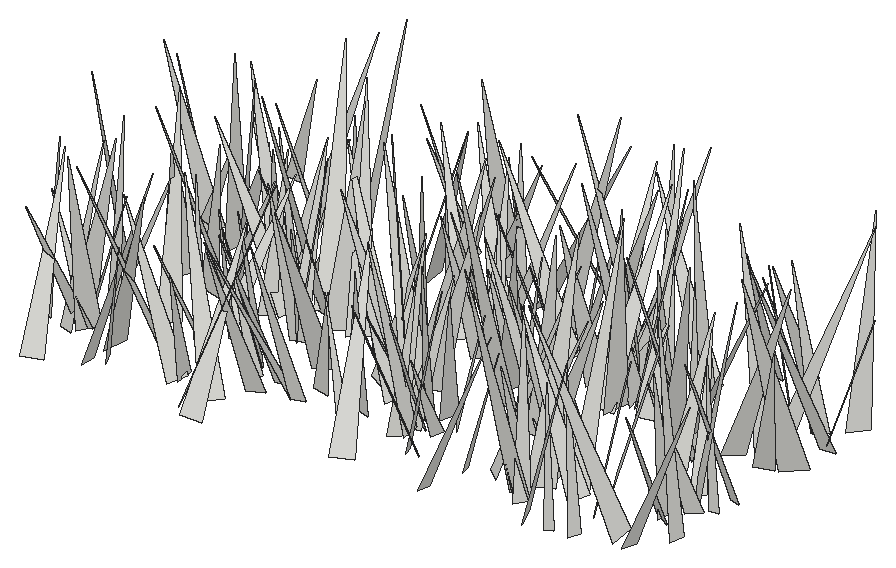
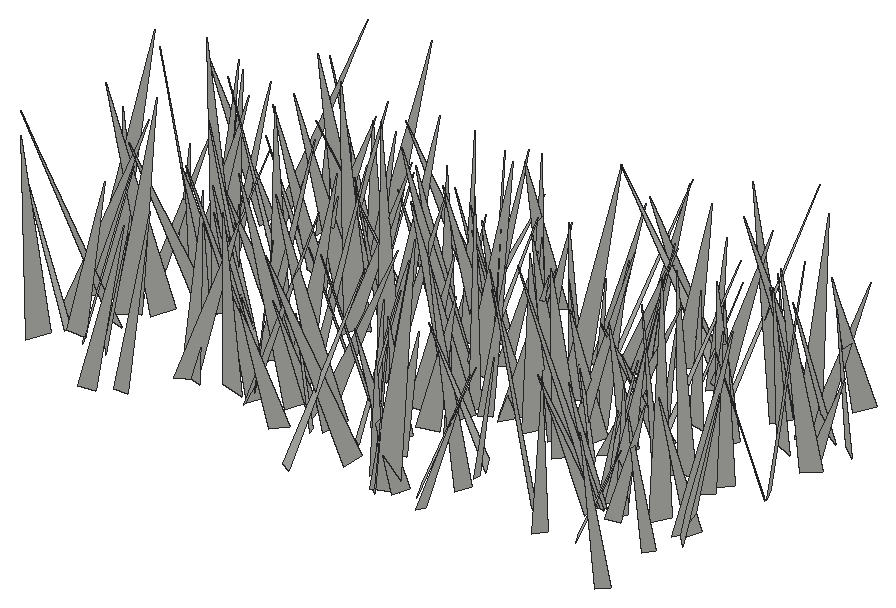
# SketchUp Ruby script. Lengths in inches.
U = 1.inch
M = Sketchup.active_model
def pt(a) = Geom::Point3d.new(a.map { |v| v * U })
def face(e, loops, mat)
  f = e.add_face(loops[0].map { |a| pt(a) })
  loops[1..].each { |l| e.add_face(l.map { |a| pt(a) }).erase! }
  f.material = f.back_material = mat if mat
  f
end
# faces: each face lists its corners as indices into pts; further lists are holes
def faces(e, pts, list, mat = nil) = list.each { |f| face(e, (f[0].is_a?(Array) ? f : [f]).map { |l| l.map { |i| pts[i] } }, mat) }
# xy, xz, yz: faces in a plane at the given z, y or x. An outline is a flat list of corners, or four numbers for a rectangle; further outlines are holes
def ring(l) = l.size == 4 ? [[l[0], l[1]], [l[2], l[1]], [l[2], l[3]], [l[0], l[3]]] : l.each_slice(2).to_a
def flat(e, list, mat, &to3) = list.each { |f| face(e, (f[0].is_a?(Array) ? f : [f]).map { |l| ring(l).map { |u, v| to3.(u, v) } }, mat) }
def xy(e, z, list, mat = nil) = flat(e, list, mat) { |x, y| [x, y, z] }
def xz(e, y, list, mat = nil) = flat(e, list, mat) { |x, z| [x, y, z] }
def yz(e, x, list, mat = nil) = flat(e, list, mat) { |y, z| [x, y, z] }
def lines(e, pts, list) = list.each { |a, b| e.add_line(pt(pts[a]), pt(pts[b])) }
# prism: a flat outline (further loops are holes) pulled along v
def prism(e, loops, v, mat = nil)
  f = face(e, loops, mat); d = Geom::Vector3d.new(v.map { |x| x * U })
  f.pushpull(f.normal.samedirection?(d) ? d.length : -d.length)
end
def box(e, o, s, mat = nil) = prism(e, [[o, [o[0] + s[0], o[1], o[2]], [o[0] + s[0], o[1] + s[1], o[2]], [o[0], o[1] + s[1], o[2]]]], [0, 0, s[2]], mat)
def at(x, y, z, deg = 0) = Geom::Transformation.translation(pt([x, y, z])) * Geom::Transformation.rotation(ORIGIN, Z_AXIS, deg.degrees)
def axes(o, x, y, z) = Geom::Transformation.new([*x, 0, *y, 0, *z, 0, *pt(o).to_a, 1])
def part(name) = M.definitions.add(name)
# library, detail: a bought-in or finely detailed component or shape, given as its bounding box
def library(name, o, s) = part(name).tap { |d| box(d.entities, o, s) }
def detail(e, o, s) = box(e.add_group.entities, o, s)
def put(e, d, t, mat = nil) = e.add_instance(d, t).tap { |i| i.material = mat if mat }
def group(e, t, mat = nil) = e.add_group.tap { |g| g.transformation = t; g.material = mat if mat }.entities
root = M.entities
c1 = part("fur_instance\#9")
p = [[0.8125,0,1.79],[0.67,-0.02,1.48],[0,-0.11,0],[0,0.11,0]]
faces(c1.entities,p,[[0,1,2,3]])
put(root,c1,axes([517.29,201.38,-21.66],[-1.69129,6.09931,0.73665],[6.01995,1.79783,-1.06428],[1.22654,-0.41345,6.23934]))
put(root,c1,axes([513.87,205.09,-21.66],[4.34393,-1.36952,0.92271],[-1.07858,-4.31928,-1.3331],[-1.25046,-1.03195,4.35524]))
put(root,c1,axes([508.99,203.98,-21.66],[3.83115,1.46002,1.29175],[1.69697,-3.89964,-0.62537],[-0.95945,-1.06731,4.05194]))
put(root,c1,axes([512.04,206.01,-21.66],[-5.96811,-4.81477,0.42538],[-4.75156,5.96808,0.88657],[0.88638,-0.42578,7.61672]))
put(root,c1,axes([505.45,201.28,-21.66],[-4.47188,4.60163,0.40246],[4.4512,4.44255,-1.33612],[1.23441,0.65071,6.27595]))
put(root,c1,axes([508.34,205.5,-21.66],[6.88515,-2.28469,0.18682],[-2.24647,-6.84269,-0.88939],[-0.45618,-0.78602,7.19959]))
put(root,c1,axes([505.62,206.01,-21.66],[0.74185,-5.118,0.35857],[-5.01336,-0.80012,-1.04825],[-1.09027,0.19676,5.06413]))
put(root,c1,axes([508.27,203.01,-21.66],[6.55283,1.12937,1.12544],[0.97488,-6.60494,0.95181],[-1.26162,0.76214,6.58096]))
put(root,c1,axes([518.27,206.27,-21.66],[1.50349,-5.86365,0.5049],[-5.82358,-1.55753,-0.74685],[-0.85041,0.2992,6.00709]))
put(root,c1,axes([540.07,204.38,-21.66],[5.73054,2.09287,1.0832],[2.24178,-5.71944,-0.8093],[-0.7265,-1.14039,6.04684]))
put(root,c1,axes([513.75,204.54,-21.66],[-5.32926,2.77314,1.19327],[2.9808,5.21718,1.1879],[0.47858,-1.6143,5.88899]))
put(root,c1,axes([505.83,206.11,-21.66],[4.78165,-4.93816,1.39024],[-4.88475,-4.96331,-0.82896],[-1.56762,0.40313,6.82367]))
put(root,c1,axes([533.17,203.42,-21.66],[5.62442,0.34622,0.61815],[0.22701,-5.5658,1.05184],[-0.67115,1.01884,5.53603]))
put(root,c1,axes([515.5625,202.65,-21.66],[6.75975,3.62956,0.52461],[3.54067,-6.74583,1.04905],[-0.95528,0.68056,7.60048]))
put(root,c1,axes([519.79,207.6,-21.66],[-4.86076,-4.47494,0.06756],[-4.36579,4.76306,1.38194],[0.98465,-0.972,6.46083]))
put(root,c1,axes([516.86,203.93,-21.66],[-4.60264,5.20733,0.96805],[5.29634,4.53648,0.77902],[0.04773,-1.24166,6.90606]))
put(root,c1,axes([545.83,206.21,-21.66],[-8.03194,-0.35365,0.82088],[-0.22203,7.97883,1.26494],[0.86581,-1.23463,7.93959]))
put(root,c1,axes([538.1,206.26,-21.66],[-1.48143,-7.59825,2.03928],[-7.84224,1.26126,-0.99758],[-0.62555,2.18232,7.67677]))
put(root,c1,axes([526.82,204.11,-21.66],[-4.67353,1.04438,0.03845],[1.02272,4.60667,-0.8165],[0.21505,0.78861,4.71868]))
put(root,c1,axes([543.59,204.51,-21.66],[-4.82421,0.67017,1.12309],[0.52178,4.9221,-0.69578],[1.19925,0.5543,4.82058]))
put(root,c1,axes([542.04,204.11,-21.66],[0.68638,4.30492,0.85677],[4.11958,-0.93113,1.37825],[-1.51508,-0.58153,4.13569]))
put(root,c1,axes([527.17,203.23,-21.66],[-3.85678,5.81728,0.33644],[5.7739,3.8696,-0.71896],[0.78484,0.11882,6.94252]))
put(root,c1,axes([530.33,206.41,-21.66],[-3.6362,-3.51378,0.23491],[-3.4583,3.49912,-1.19165],[-0.6648,1.01649,4.91412]))
put(root,c1,axes([520.81,207.0625,-21.66],[-0.18696,-5.47828,1.21386],[-5.53827,-0.01495,-0.92048],[-0.90141,1.22808,5.40363]))
put(root,c1,axes([546.94,205.55,-21.66],[5.55155,-0.72144,0.45458],[-0.77671,-5.51397,0.73462],[-0.35191,0.78896,5.54982]))
put(root,c1,axes([513.29,207.97,-21.66],[-3.4189,-2.83051,0.24342],[-2.77437,3.40847,0.66713],[0.61145,-0.36118,4.38812]))
put(root,c1,axes([537.24,207.9375,-21.66],[4.28198,-1.79299,1.3249],[-1.43721,-4.41332,-1.32759],[-1.70429,-0.78312,4.44833]))
put(root,c1,axes([537.33,206.62,-21.66],[-3.51582,-2.14374,0.80605],[-2.26912,3.46073,-0.69338],[0.31056,1.01688,4.05904]))
put(root,c1,axes([524.47,208.31,-21.66],[-0.27546,-6.0552,1.07535],[-6.00995,0.49341,1.23885],[1.30474,0.99438,5.93351]))
put(root,c1,axes([502.96,205.89,-21.66],[2.73063,4.59292,1.67983],[4.59916,-3.06583,0.90635],[-1.66266,-0.93747,5.2659]))
put(root,c1,axes([538.68,205.75,-21.66],[-5.6137,1.8249,1.28834],[1.63706,5.7317,-0.98561],[1.51991,0.56669,5.82001]))
put(root,c1,axes([517.29,207.57,-21.66],[-3.50463,1.38607,1.3282],[1.66931,3.56562,0.68373],[0.94799,-1.15452,3.70623]))
put(root,c1,axes([504.88,205.18,-21.66],[2.36342,5.34352,0.74133],[5.25737,-2.46286,0.99138],[-1.20944,-0.26392,5.75813]))
put(root,c1,axes([504.83,207.71,-21.66],[4.88196,1.64498,0.71636],[1.77456,-4.73338,-1.22423],[-0.26474,-1.39349,5.00407]))
put(root,c1,axes([546.35,209.35,-21.66],[-1.70648,-4.83175,0.15849],[-4.67215,1.69151,1.26205],[1.24174,-0.27565,4.96639]))
put(root,c1,axes([518.73,207.97,-21.66],[-1.8038,-4.78632,0.84713],[-4.75617,1.55162,-1.36069],[-1.00264,1.25053,4.93062]))
put(root,c1,axes([529.75,208.97,-21.66],[2.79879,-2.29313,0.37979],[-2.08936,-2.74248,-1.16161],[-1.01846,-0.6755,3.42672]))
put(root,c1,axes([533.73,206.61,-21.66],[3.61402,1.40651,0.81578],[1.29809,-3.69316,0.61679],[-0.97915,0.29527,3.8287]))
put(root,c1,axes([528.375,208.27,-21.66],[-6.31827,-0.38458,1.65434],[-0.20418,6.49842,0.73085],[1.68614,-0.65417,6.28763]))
put(root,c1,axes([521.23,208.6875,-21.66],[0.93641,-4.49496,0.58968],[-4.44892,-0.79539,1.00188],[0.87152,0.76939,4.48082]))
put(root,c1,axes([529.68,206.29,-21.66],[4.20978,2.5999,1.29958],[2.36123,-4.39284,1.13935],[-1.69498,0.33775,4.81493]))
put(root,c1,axes([528.42,209.24,-21.66],[-1.9531,-3.93926,0.49775],[-3.87343,2.01224,0.72636],[0.87298,0.11511,4.33645]))
put(root,c1,axes([516.32,209.37,-21.66],[-3.7934,-3.57067,0.95546],[-3.47781,3.9116,0.81037],[1.25196,0.04698,5.14615]))
put(root,c1,axes([541.03,208.16,-21.66],[-5.49496,2.98551,0.84144],[3.09795,5.36781,1.18541],[0.15494,-1.44541,6.14025]))
put(root,c1,axes([528.74,209.5,-21.66],[-1.97091,-5.99186,1.73382],[-5.97714,2.33419,1.27215],[1.7839,1.20092,6.17807]))
put(root,c1,axes([503.9,208.01,-21.66],[-1.40668,3.30295,0.84871],[3.29754,1.08331,1.24951],[-0.86952,-1.23511,3.36556]))
put(root,c1,axes([519.7,210.99,-21.66],[2.52782,-6.77606,0.30453],[-6.73549,-2.54598,-0.74076],[-0.80053,0.02468,7.19418]))
put(root,c1,axes([527.9,207.28,-21.66],[3.76541,-0.98312,2.37268],[-1.72485,-4.08783,1.04352],[-1.9029,1.75998,3.74912]))
put(root,c1,axes([503.2,209.0625,-21.66],[2.93008,-5.46925,1.49234],[-5.65269,-2.69042,1.23848],[0.43226,1.89052,6.07982]))
put(root,c1,axes([546.32,209.79,-21.66],[5.03393,-2.19184,1.50174],[-1.99616,-5.24318,-0.96135],[-1.75349,-0.32355,5.40559]))
put(root,c1,axes([543.01,207.18,-21.66],[3.77893,2.89431,1.05154],[2.64296,-3.90266,1.24382],[-1.58036,0.3941,4.59459]))
put(root,c1,axes([538.375,210.07,-21.66],[-6.39849,-1.36399,1.46981],[-1.16574,6.52941,0.98452],[1.63152,-0.68393,6.46776]))
put(root,c1,axes([526.34,211.04,-21.66],[-3.05725,-3.63504,0.09512],[-3.51202,2.98398,1.15363],[0.94245,-0.67208,4.60753]))
put(root,c1,axes([548.6,207.93,-21.66],[-7.01031,-0.43579,1.43561],[-0.72042,6.99511,-1.39453],[1.31601,1.50792,6.88401]))
put(root,c1,axes([506.15,208.04,-21.66],[1.54209,5.92638,1.72605],[6.04197,-1.81335,0.82809],[-1.2633,-1.43843,6.06748]))
put(root,c1,axes([538.4,207.82,-21.66],[-4.94866,6.16749,2.69055],[6.18584,5.48419,-1.19385],[2.6481,-1.28527,7.81677]))
put(root,c1,axes([528.09,208.59,-21.66],[-2.58112,4.19595,2.18678],[4.13957,3.20902,-1.27135],[2.29171,-1.07069,4.75939]))
put(root,c1,axes([547.41,211.04,-21.66],[1.87791,-4.76016,0.94457],[-4.63856,-2.05833,-1.15104],[-1.42657,0.4266,4.98606]))
put(root,c1,axes([528.99,211.04,-21.66],[4.92449,-2.5321,0.51516],[-2.43841,-4.92066,-0.87679],[-0.85503,-0.55051,5.46748]))
put(root,c1,axes([522.125,210.79,-21.66],[0.84886,-4.32385,0.54485],[-4.30912,-0.7498,0.76315],[0.65118,0.6747,4.3398]))
put(root,c1,axes([511.91,209.07,-21.66],[-0.00345,4.9845,1.60202],[5.18158,-0.22632,0.71534],[-0.75028,-1.58596,4.93291]))
put(root,c1,axes([535.35,207.25,-21.66],[4.61833,5.37447,0.17353],[5.34108,-4.61135,0.67253],[-0.62281,0.30742,7.05419]))
put(root,c1,axes([527.52,208.28,-21.66],[0.92539,5.82013,0.73982],[5.78512,-1.02986,0.86568],[-0.97656,-0.58571,5.82931]))
put(root,c1,axes([530.06,210.43,-21.66],[3.37975,2.64749,1.02841],[2.82915,-3.2791,-0.85611],[-0.25046,-1.31446,4.20701]))
put(root,c1,axes([539.36,210.16,-21.66],[-2.08975,2.94897,0.92989],[3.09202,1.98432,0.65582],[-0.0238,-1.13764,3.55435]))
put(root,c1,axes([525.2,210.48,-21.66],[-3.9914,1.89648,0.82188],[2.01712,3.964,0.64912],[0.45094,-0.94526,4.3711]))
put(root,c1,axes([536.39,210.77,-21.66],[5.35038,-4.23141,0.69897],[-4.27634,-5.17862,1.38378],[0.32603,1.51562,6.67957]))
put(root,c1,axes([513.27,210.33,-21.66],[-1.82115,-3.36265,1.61921],[-3.73204,1.65736,-0.7556],[0.03439,1.7865,3.74875]))
put(root,c1,axes([515.16,210.56,-21.66],[-1.86227,-3.58892,1.59018],[-3.91628,1.57852,-1.02377],[-0.26793,1.87217,3.91156]))
put(root,c1,axes([541.4375,211.08,-21.66],[5.88028,2.97965,0.94292],[3.11911,-5.72141,-1.37172],[-0.19635,-1.65292,6.44782]))
put(root,c1,axes([503.45,212.76,-21.66],[-6.01698,-4.0059,2.23214],[-3.85326,6.41302,1.12219],[2.48637,0.24439,7.14087]))
put(root,c1,axes([511.94,212.45,-21.66],[-5.99234,-4.15881,0.58341],[-4.19764,5.96205,-0.6148],[0.12593,0.83815,7.26814]))
put(root,c1,axes([509.05,209.68,-21.66],[-5.83364,4.02968,1.05878],[3.90844,5.92385,-1.01134],[1.44341,0.24573,7.01761]))
put(root,c1,axes([534.62,212.49,-21.66],[2.7668,-7.06079,2.0724],[-7.35623,-2.5972,0.97226],[0.18857,2.28135,7.52095]))
put(root,c1,axes([516.43,212.6,-21.66],[0.40641,-5.35004,1.66525],[-5.54368,-0.62666,-0.66032],[-0.81458,1.59547,5.32467]))
put(root,c1,axes([516.32,213.1,-21.66],[4.42301,-0.66017,1.25029],[-0.31732,-4.46498,-1.23502],[-1.37781,-1.09094,4.29808]))
put(root,c1,axes([540.4,208.84,-21.66],[0.71123,8.26754,0.30404],[8.18462,-0.74766,1.1847],[-1.20692,-0.19821,8.21307]))
put(root,c1,axes([523.04,211.72,-21.66],[2.00403,4.77087,1.2081],[4.88814,-1.77806,-1.08691],[0.57161,-1.52123,5.05925]))
put(root,c1,axes([534.01,210.9375,-21.66],[2.59525,5.12132,1.23508],[5.09738,-2.78884,0.85303],[-1.33041,-0.69505,5.67763]))
put(root,c1,axes([506.05,213.63,-21.66],[5.02867,-2.50397,0.95955],[-2.41233,-5.11484,-0.70513],[-1.17101,-0.21602,5.57317]))
put(root,c1,axes([534.87,212.95,-21.66],[-6.53044,0.59698,0.86107],[0.69842,6.53195,0.76827],[0.78105,-0.84949,6.51251]))
put(root,c1,axes([525.59,212.25,-21.66],[-4.55755,6.1935,2.40469],[6.62517,4.45559,1.08074],[0.49905,-2.58872,7.61332]))
put(root,c1,axes([524.87,212.16,-21.66],[-5.85102,-5.01294,3.05498],[-5.59861,6.06235,-0.77491],[1.76582,2.61061,7.66574]))
put(root,c1,axes([546.52,212.41,-21.66],[-3.91032,-4.73518,3.93684],[-5.20514,5.03349,0.88414],[3.29046,2.33522,6.07707]))
put(root,c1,axes([548.22,211.85,-21.66],[0.93593,4.40998,1.37185],[4.37962,-1.29175,1.16453],[-1.46587,-1.0437,4.3552]))
put(root,c1,axes([548.48,213.51,-21.66],[-2.25031,-4.2676,0.76277],[-4.32128,2.13921,-0.77999],[-0.34742,1.03417,4.76108]))
put(root,c1,axes([508.67,213.96,-21.66],[0.4901,-6.09421,1.40714],[-6.12992,-0.18765,1.32232],[1.24239,1.47818,5.96918]))
put(root,c1,axes([530.84,214.09,-21.66],[-1.51779,-7.89387,2.17922],[-8.18213,1.37007,-0.73587],[-0.33897,2.275,8.00471]))
put(root,c1,axes([526.27,212.98,-21.66],[4.89354,-4.52263,1.72188],[-4.82903,-4.72322,1.31813],[-0.31551,2.14541,6.53173]))
put(root,c1,axes([529.74,215.57,-21.66],[6.8807,-3.2851,0.24825],[-3.20439,-6.80705,-1.26238],[-0.76512,-1.03432,7.51946]))
put(root,c1,axes([503.4,213.29,-21.66],[3.56732,3.05528,0.6125],[3.0981,-3.37772,-1.19517],[0.33415,-1.30074,4.54225]))
put(root,c1,axes([511.95,211.6,-21.66],[-0.74484,5.04348,0.31723],[4.84937,0.80355,-1.38926],[1.42161,-0.09859,4.90524]))
put(root,c1,axes([506.35,214.9375,-21.66],[4.04472,-2.80495,1.23292],[-2.68281,-4.22845,-0.81868],[-1.47998,-0.00072,4.85358]))
put(root,c1,axes([525.9,213.25,-21.66],[7.69259,-0.4984,1.40276],[-0.64413,-7.77059,0.77146],[-1.3421,0.87272,7.67002]))
put(root,c1,axes([541.98,215.56,-21.66],[7.73764,-3.02475,0.93063],[-2.93122,-7.77665,-0.90436],[-1.19293,-0.51074,8.25847]))
put(root,c1,axes([534.57,216.1,-21.66],[-3.08937,-5.14938,0.76665],[-5.09175,3.1744,0.80332],[1.08532,0.23487,5.95105]))
put(root,c1,axes([522.34,215.84,-21.66],[3.93846,-2.19121,0.70559],[-1.95473,-3.92185,-1.26841],[-1.21585,-0.79274,4.32481]))
put(root,c1,axes([529.62,215.72,-21.66],[-2.67742,-5.68655,1.10676],[-5.79247,2.6077,-0.61446],[-0.09527,1.2623,6.25523]))
put(root,c1,axes([546.22,212.88,-21.66],[-4.08982,2.78235,0.32679],[2.66533,4.04258,-1.06229],[0.86271,0.7007,4.83111]))
put(root,c1,axes([513.89,214.9,-21.66],[-6.12139,2.10353,0.29479],[2.12072,6.0019,1.20952],[-0.1196,-1.23917,6.35872]))
put(root,c1,axes([521.13,215.43,-21.66],[-5.2528,1.04607,1.18822],[1.28573,5.22141,1.0871],[0.92359,-1.31932,5.24446]))
put(root,c1,axes([523.26,215.64,-21.66],[6.36794,0.62079,2.33056],[0.97414,-6.68136,-0.88201],[-2.20634,-1.15823,6.33704]))
put(root,c1,axes([513.05,213.86,-21.66],[-4.28711,2.60894,1.39768],[2.40918,4.50508,-1.01958],[1.71929,0.19268,4.91389]))
put(root,c1,axes([509.375,214.49,-21.66],[3.95352,-1.35205,0.74696],[-1.51739,-3.78343,1.18299],[-0.28899,1.3689,4.00736]))
put(root,c1,axes([515.64,216.04,-21.66],[-3.53449,-6.31522,1.62159],[-6.50822,3.306,-1.31053],[-0.39309,2.04757,7.11738]))
put(root,c1,axes([533,215.34,-21.66],[2.4928,2.63766,0.46244],[2.65596,-2.35455,-0.88721],[0.34203,-0.94022,3.51911]))
put(root,c1,axes([542.6,216.67,-21.66],[-3.61548,-1.81279,0.7212],[-1.71327,3.67656,0.65243],[0.9333,-0.2734,3.99152]))
put(root,c1,axes([529.875,216.3125,-21.66],[0.54062,-3.9189,1.26852],[-4.01221,-0.79056,-0.73238],[-0.93225,1.12979,3.88763]))
put(root,c1,axes([515.33,213.99,-21.66],[-4.48164,3.41054,1.04148],[3.17852,4.57879,-1.31654],[1.61662,0.45221,5.47573]))
put(root,c1,axes([543.35,214.53,-21.66],[-2.74828,4.07366,1.32335],[3.94461,3.01992,-1.10419],[1.66916,-0.42944,4.78838]))
put(root,c1,axes([521.12,214.92,-21.66],[-5.13567,3.95215,0.39173],[3.97037,5.09374,0.66187],[-0.09557,-0.76314,6.44644]))
put(root,c1,axes([513.79,216.36,-21.66],[4.93042,2.67254,1.54888],[2.99605,-4.84755,-1.1728],[-0.75178,-1.79146,5.48417]))
put(root,c1,axes([543.22,216.17,-21.66],[-5.70122,-3.26457,0.62497],[-3.32356,5.6155,-0.98593],[0.04408,1.16649,6.49533]))
put(root,c1,axes([548.85,218.66,-21.66],[4.03591,-7.21522,0.98619],[-7.10178,-4.1491,-1.2924],[-1.61145,0.21471,8.16564]))
put(root,c1,axes([547.27,217.75,-21.66],[2.80299,-5.03768,0.10257],[-5.00094,-2.76705,0.76127],[0.6159,0.45904,5.71449]))
put(root,c1,axes([517.29,215.02,-21.66],[5.828,-3.21448,3.45143],[-4.0564,-6.21538,1.06086],[-2.40642,2.69201,6.57061]))
put(root,c1,axes([526.02,217.65,-21.66],[1.56838,-4.91392,1.31708],[-4.91027,-1.82266,-0.95305],[-1.33063,0.93404,5.06933]))
put(root,c1,axes([509.39,215.86,-21.66],[-5.60874,-1.91132,2.91151],[-2.48414,6.06379,-0.80475],[2.44113,1.77916,5.87056]))
put(root,c1,axes([536.06,217.88,-21.66],[7.26083,-2.43104,1.92439],[-2.31077,-7.51014,-0.76873],[-2.06726,-0.14373,7.61831]))
put(root,c1,axes([523.2,216.86,-21.66],[5.70203,-3.94241,1.833],[-4.2894,-5.59456,1.31056],[-0.70959,2.13867,6.80721]))
put(root,c1,axes([518.92,215.28,-21.66],[5.10712,-2.96498,5.20518],[-4.57955,-6.3419,0.88079],[-3.86171,3.59957,5.83935]))
put(root,c1,axes([544.84,217.92,-21.66],[6.03076,-3.95506,0.64167],[-4.00583,-5.92637,1.12057],[0.08689,1.28836,7.12438]))
put(root,c1,axes([533.49,219.43,-21.66],[3.60817,-5.34608,1.25489],[-5.24687,-3.79935,-1.09972],[-1.62036,0.39817,6.35531]))
put(root,c1,axes([510.59,219.62,-21.66],[-2.24525,-3.81491,0.32062],[-3.67914,2.25292,1.04201],[1.05843,-0.26136,4.3022]))
put(root,c1,axes([506.52,219.09,-21.66],[7.00851,-2.19777,2.01204],[-2.01969,-7.2848,-0.92211],[-2.19075,-0.31499,7.28692]))
put(root,c1,axes([542.125,216.87,-21.66],[6.26365,0.83218,0.34032],[0.77044,-6.2027,0.98722],[-0.46342,0.93576,6.24109]))
put(root,c1,axes([542.62,216.94,-21.66],[-4.924,0.48292,1.1816],[0.20052,4.94285,-1.18453],[1.26062,1.10005,4.80373]))
put(root,c1,axes([536.34,219.5,-21.66],[-7.391,-1.41623,2.02124],[-1.14457,7.62073,1.15434],[2.18657,-0.79801,7.4364]))
put(root,c1,axes([504.47,219.6875,-21.66],[-6.49711,1.14641,2.18071],[1.63194,6.61021,1.38712],[1.84567,-1.80917,6.45001]))
put(root,c1,axes([515.51,216.64,-21.66],[-5.56313,6.05819,1.00831],[6.02083,5.64819,-0.71719],[1.2116,-0.25113,8.19364]))
put(root,c1,axes([503.92,219.2,-21.66],[3.45367,-2.54495,0.42724],[-2.57712,-3.36456,0.79082],[0.1334,0.88889,4.21654]))
put(root,c1,axes([546.35,219.4,-21.66],[-5.45216,4.70878,2.71596],[5.23215,5.58914,0.81316],[1.47433,-2.42158,7.15803]))
put(root,c1,axes([512.55,218.59,-21.66],[3.9235,0.14114,0.37721],[0.06723,-3.8717,0.74932],[-0.3971,0.73898,3.85386]))
put(root,c1,axes([508.625,220.15,-21.66],[3.85883,-1.0172,1.02296],[-0.87371,-3.97244,-0.65425],[-1.14794,-0.39587,3.93665]))
put(root,c1,axes([526.52,220.89,-21.66],[-0.43336,-3.79274,0.22877],[-3.61563,0.48241,1.14868],[1.16807,0.08612,3.64049]))
put(root,c1,axes([536.4,219.5,-21.66],[7.04246,3.4796,1.7186],[3.70112,-7.09298,-0.80545],[-1.16744,-1.49647,7.81378]))
put(root,c1,axes([509.68,219.33,-21.66],[-3.34146,5.15286,1.47209],[5.35695,3.16362,1.08579],[-0.14849,-1.82317,6.0447]))
put(root,c1,axes([535.42,217.35,-21.66],[-1.59566,7.05244,0.57454],[6.94745,1.67322,-1.24356],[1.34162,-0.27674,7.12297]))
put(root,c1,axes([548.9,221.69,-21.66],[-1.75901,-6.72397,0.92553],[-6.70142,1.56883,-1.33876],[-1.07676,1.22044,6.82009]))
put(root,c1,axes([510.99,219,-21.66],[-4.31173,0.11749,0.33288],[0.02447,4.16916,-1.1546],[0.35215,1.14887,4.15592]))
put(root,c1,axes([504.12,220.18,-21.66],[-4.01169,-3.78695,1.3287],[-4.00574,3.89344,-0.9976],[0.2459,1.64323,5.42581]))
put(root,c1,axes([536.8,221.62,-21.66],[4.83805,-1.95602,0.87332],[-1.75837,-4.85831,-1.14034],[-1.22345,-0.75248,5.09238]))
put(root,c1,axes([522.14,219.69,-21.66],[-3.8319,-0.08961,1.0116],[-0.27638,3.8917,-0.7022],[0.97723,0.7493,3.76807]))
put(root,c1,axes([524.01,219.13,-21.66],[-3.78417,5.30239,0.2634],[5.25954,3.70033,1.07214],[-0.72248,-0.83479,6.42541]))
put(root,c1,axes([510.1875,220.1875,-21.66],[0.83525,-3.69964,2.10924],[-4.22949,-0.46947,0.8514],[0.49764,2.21949,3.69595]))
put(root,c1,axes([508.67,220.91,-21.66],[-2.76713,3.18046,1.2921],[3.43249,2.58898,0.97827],[0.05304,-1.61979,4.10065]))
put(root,c1,axes([534.81,221.82,-21.66],[3.60771,1.96245,2.32029],[2.67745,-3.75626,-0.98607],[-1.43745,-2.07119,3.98679]))
put(root,c1,axes([518.16,221.82,-21.66],[-3.2792,-1.26365,1.37089],[-0.97388,3.52607,0.9207],[1.58988,-0.44645,3.3915]))
put(root,c1,axes([530.21,220.93,-21.66],[-6.66331,2.16551,0.21128],[2.17487,6.60915,0.85019],[-0.06344,-0.87375,6.95459]))
put(root,c1,axes([526.24,222.98,-21.66],[-3.04266,-3.74721,0.50143],[-3.60797,3.07034,1.05183],[1.12942,-0.28668,4.71094]))
put(root,c1,axes([538.24,218.08,-21.66],[0.0768,8.17284,0.16546],[8.06568,-0.10268,1.32775],[-1.3295,-0.15078,8.06464]))
put(root,c1,axes([510.43,220.11,-21.66],[4.03025,7.20792,1.49357],[7.34455,-3.82368,-1.36555],[0.49235,-1.96292,8.14446]))
put(root,c1,axes([504.72,222.46,-21.66],[1.3305,-3.93215,0.09517],[-3.71952,-1.22514,1.38031],[1.27907,0.52755,3.91494]))
put(root,c1,axes([531.71,221.72,-21.66],[6.48225,-3.39085,0.68777],[-3.4557,-6.41712,0.9323],[-0.17042,1.14593,7.25591]))
put(root,c1,axes([525.15,220.43,-21.66],[-0.19051,3.61425,0.52762],[3.57644,0.0773,0.76192],[-0.74175,-0.55561,3.53816]))
put(root,c1,axes([534.33,221.57,-21.66],[1.01992,4.1189,1.46608],[4.23417,-0.55549,-1.38501],[1.0893,-1.69737,4.0109]))
put(root,c1,axes([510.3,220.9,-21.66],[3.86814,-0.78573,1.02615],[-1.07279,-3.75781,1.16655],[-0.72076,1.37634,3.77081]))
put(root,c1,axes([546.43,223.43,-21.66],[-4.48519,-3.52054,0.94744],[-3.42145,4.58335,0.83384],[1.25916,-0.08621,5.64055]))
put(root,c1,axes([518.52,220.39,-21.66],[4.75922,3.00167,0.77273],[2.8511,-4.79497,1.06623],[-1.21588,0.50555,5.5248]))
put(root,c1,axes([517.86,223.44,-21.66],[6.9866,-0.46387,0.39437],[-0.38095,-6.874,-1.33651],[-0.47495,-1.31005,6.87325]))
put(root,c1,axes([524.48,220.81,-21.66],[-3.96377,3.38106,0.80717],[3.27975,4.04327,-0.83051],[1.15166,0.12228,5.14327]))
put(root,c1,axes([533.98,222.63,-21.66],[4.85202,-3.37562,1.03104],[-3.52041,-4.75453,1.00059],[-0.25408,1.41409,5.82544]))
put(root,c1,axes([546.23,220.7,-21.66],[3.64323,6.95762,0.66244],[6.95502,-3.53547,-1.11744],[0.68929,-1.10109,7.77386]))
put(root,c1,axes([548.1,222.89,-21.66],[4.88732,1.92922,0.49219],[1.99044,-4.76555,-1.08522],[-0.04774,-1.19066,5.14102]))
put(root,c1,axes([524.73,222.1875,-21.66],[4.20289,4.66758,0.96744],[4.74909,-3.98911,-1.38552],[0.41036,-1.63927,6.12625]))
put(root,c1,axes([534.64,221.13,-21.66],[3.51205,7.24819,1.1392],[7.33442,-3.43356,-0.76524],[0.20101,-1.35755,8.01781]))
put(root,c1,axes([534.61,222.52,-21.66],[-7.94923,-1.56442,0.5472],[-1.62855,7.87073,-1.15603],[0.30767,1.24144,8.0188]))
put(root,c1,axes([547.24,223.1,-21.66],[0.3865,-5.10308,2.42648],[-5.49086,-0.91339,-1.04632],[-1.33405,2.28099,5.00959]))
put(root,c1,axes([529.2,223.54,-21.66],[3.2608,1.42212,0.87051],[1.60342,-3.19897,-0.78016],[-0.45742,-1.07574,3.47082]))
put(root,c1,axes([530.23,221.98,-21.66],[4.26964,0.47793,1.18834],[0.14194,-4.28676,1.21405],[-1.27296,1.12502,4.1212]))
put(root,c1,axes([528.43,222.31,-21.66],[7.3545,-2.24014,2.18394],[-2.66673,-7.40612,1.38362],[-1.63595,2.00191,7.56257]))
put(root,c1,axes([538.65,223.09,-21.66],[-1.16984,-6.03511,2.92768],[-6.70455,0.96018,-0.69968],[-0.2073,3.00298,6.1075]))
put(root,c1,axes([538.87,223.27,-21.66],[-5.22041,4.31379,0.87725],[4.39805,5.05275,1.32586],[-0.18846,-1.57859,6.64105]))
put(root,c1,axes([512.71,223.14,-21.66],[4.94057,6.27292,2.28459],[6.62263,-4.9638,-0.69253],[-0.84236,-2.23369,7.95482]))
put(root,c1,axes([511.12,224.6875,-21.66],[4.3252,-1.84495,1.08949],[-1.74272,-4.45705,-0.62914],[-1.2465,-0.1704,4.65998]))
put(root,c1,axes([523.49,222.79,-21.66],[-3.54308,4.52564,0.44169],[4.5332,3.47169,0.79207],[-0.35583,-0.83417,5.69276]))
put(root,c1,axes([544.8,223.41,-21.66],[-3.71707,-2.68533,1.32909],[-2.9797,3.53518,-1.19076],[0.31439,1.75658,4.42828]))
put(root,c1,axes([509.03,223.78,-21.66],[-3.56795,-1.90054,0.20659],[-1.88749,3.43261,-1.0196],[-0.30353,0.99505,3.91187]))
put(root,c1,axes([535.87,222.65,-21.66],[0.42916,7.00561,1.64499],[7.11073,-0.66598,0.98114],[-1.10544,-1.56418,6.94983]))
put(root,c1,axes([521.37,226.44,-21.66],[4.41778,-6.32124,1.65754],[-6.32459,-4.6393,-0.83587],[-1.6447,0.86086,7.66656]))
put(root,c1,axes([540.92,226.83,-21.66],[-0.50575,-5.47671,0.42869],[-5.44927,0.55465,0.65709],[0.69543,0.36321,5.46062]))
put(root,c1,axes([527.65,227.89,-21.66],[-3.98509,-5.15803,0.00595],[-5.07141,3.91953,1.18509],[0.94137,-0.71992,6.40951]))
put(root,c1,axes([519.8,225.21,-21.66],[-5.05494,-2.22544,0.30278],[-2.23904,4.935,-1.10864],[-0.17591,1.1357,5.41072]))
put(root,c1,axes([525.05,224.88,-21.66],[6.85637,-0.90607,0.05149],[-0.90407,-6.7849,0.99057],[0.07926,0.98874,6.84468]))
put(root,c1,axes([548.83,224.69,-21.66],[5.64429,-3.09602,3.33103],[-3.78051,-6.14532,0.69416],[-2.52761,2.27789,6.40012]))
put(root,c1,axes([520.56,225.97,-21.66],[4.45339,-2.56263,0.11815],[-2.55046,-4.39735,0.75645],[0.27609,0.71411,5.08208]))
put(root,c1,axes([518.36,226.82,-21.66],[-4.47409,-0.55232,0.95951],[-0.288,4.43762,1.21151],[1.069,-1.11608,4.34221]))
put(root,c1,axes([521.87,226.88,-21.66],[-2.90046,-3.39812,1.38689],[-3.27993,3.19309,0.96417],[1.64705,0.37459,4.36237]))
put(root,c1,axes([523.17,224.98,-21.66],[-4.45117,0.87592,1.04433],[0.68712,4.52233,-0.86441],[1.17717,0.67238,4.45342]))
put(root,c1,axes([542.72,227.79,-21.66],[2.25117,-4.50739,0.41367],[-4.42833,-2.28883,-0.84056],[-0.93676,-0.01195,4.96767]))
put(root,c1,axes([530.92,224.43,-21.66],[-2.87102,4.68172,0.40163],[4.57171,2.89185,-1.02921],[1.08596,0.20316,5.39463]))
put(root,c1,axes([504.1,227.58,-21.66],[1.4923,-4.43759,0.64343],[-4.35505,-1.27294,1.3215],[1.06759,1.01025,4.49142]))
